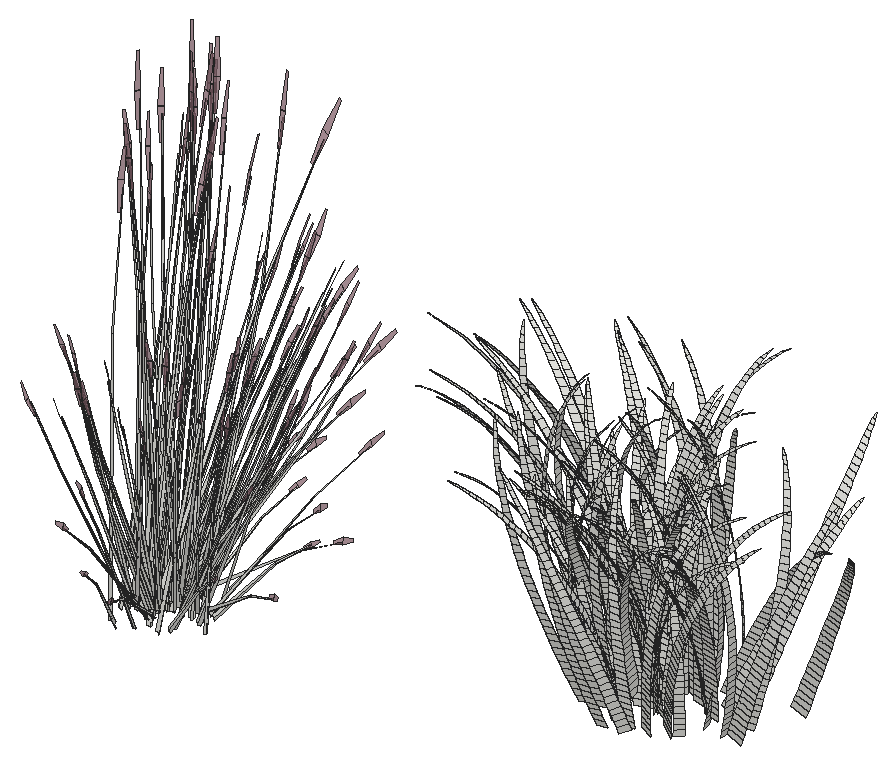
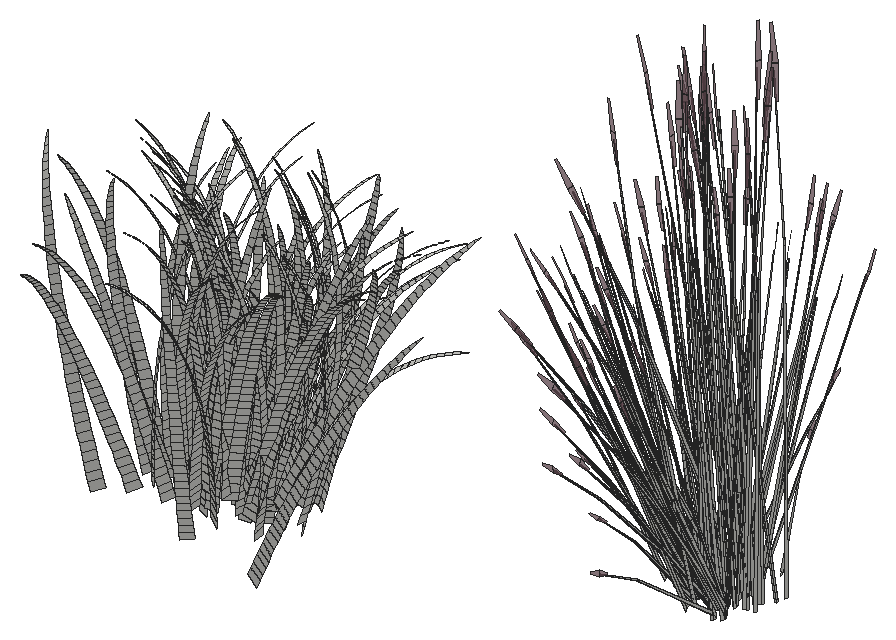
# SketchUp Ruby script. Lengths in inches.
U = 1.inch
M = Sketchup.active_model
def pt(a) = Geom::Point3d.new(a.map { |v| v * U })
def face(e, loops, mat)
  f = e.add_face(loops[0].map { |a| pt(a) })
  loops[1..].each { |l| e.add_face(l.map { |a| pt(a) }).erase! }
  f.material = f.back_material = mat if mat
  f
end
# faces: each face lists its corners as indices into pts; further lists are holes
def faces(e, pts, list, mat = nil) = list.each { |f| face(e, (f[0].is_a?(Array) ? f : [f]).map { |l| l.map { |i| pts[i] } }, mat) }
# xy, xz, yz: faces in a plane at the given z, y or x. An outline is a flat list of corners, or four numbers for a rectangle; further outlines are holes
def ring(l) = l.size == 4 ? [[l[0], l[1]], [l[2], l[1]], [l[2], l[3]], [l[0], l[3]]] : l.each_slice(2).to_a
def flat(e, list, mat, &to3) = list.each { |f| face(e, (f[0].is_a?(Array) ? f : [f]).map { |l| ring(l).map { |u, v| to3.(u, v) } }, mat) }
def xy(e, z, list, mat = nil) = flat(e, list, mat) { |x, y| [x, y, z] }
def xz(e, y, list, mat = nil) = flat(e, list, mat) { |x, z| [x, y, z] }
def yz(e, x, list, mat = nil) = flat(e, list, mat) { |y, z| [x, y, z] }
def lines(e, pts, list) = list.each { |a, b| e.add_line(pt(pts[a]), pt(pts[b])) }
# prism: a flat outline (further loops are holes) pulled along v
def prism(e, loops, v, mat = nil)
  f = face(e, loops, mat); d = Geom::Vector3d.new(v.map { |x| x * U })
  f.pushpull(f.normal.samedirection?(d) ? d.length : -d.length)
end
def box(e, o, s, mat = nil) = prism(e, [[o, [o[0] + s[0], o[1], o[2]], [o[0] + s[0], o[1] + s[1], o[2]], [o[0], o[1] + s[1], o[2]]]], [0, 0, s[2]], mat)
def at(x, y, z, deg = 0) = Geom::Transformation.translation(pt([x, y, z])) * Geom::Transformation.rotation(ORIGIN, Z_AXIS, deg.degrees)
def axes(o, x, y, z) = Geom::Transformation.new([*x, 0, *y, 0, *z, 0, *pt(o).to_a, 1])
def part(name) = M.definitions.add(name)
# library, detail: a bought-in or finely detailed component or shape, given as its bounding box
def library(name, o, s) = part(name).tap { |d| box(d.entities, o, s) }
def detail(e, o, s) = box(e.add_group.entities, o, s)
def put(e, d, t, mat = nil) = e.add_instance(d, t).tap { |i| i.material = mat if mat }
def group(e, t, mat = nil) = e.add_group.tap { |g| g.transformation = t; g.material = mat if mat }.entities
root = M.entities
M.materials.add("LightPink_Translucent").color = [144, 107, 117]
M.materials["LightPink_Translucent"].alpha = 0.75
c1 = part("blade")
p = [[2.15,0.21,22],[0,0.17,0],[0.09,0.45,0],[2.18,0.31,22],[2.29,0.31,22],[0.38,0.45,0],
  [2.48,0.24,33],[2.49,0.24,33],[2.48,0.22,33]]
faces(c1.entities,p,[[0,1,2,3],[4,5,2,3],[6,3,4,7],[8,0,3,6]])
c2 = part("seeds")
p = [[0.3,-0.1,1.38],[-0.01,-0.03,1.59],[-0.01,-0.03,0.03],[0.14,-0.07,-0.07],[0.29,-0.03,3],[0.15,0.01,3.11]]
faces(c2.entities,p,[[0,1,2,3],[1,0,4,5]],"LightPink_Translucent")
c3 = part("blade with seeds")
put(c3.entities,c1,at(0,0,0))
put(c3.entities,c2,axes([2.4,0.25,30.99],[1.5799,-0.05474,1.17369],[-0.12525,1.92788,0.29478],[-0.07173,-0.02425,1.56792]))
c4 = part("fur_instance\#8")
p = [[-0.25,1.49,0.03],[0.25,-1.49,-0.03],[0.44,-1.47,1.51],[-0.05,1.47,1.57],[0.65,-1.44,3.05],[0.16,1.45,3.11],
  [0.86,-1.42,4.59],[0.38,1.44,4.65],[1.1,-1.39,6.13],[0.62,1.43,6.18],[1.34,-1.35,7.66],[0.875,1.42,7.72],
  [1.6,-1.32,9.19],[1.14,1.41,9.25],[1.88,-1.28,10.72],[1.43,1.41,10.78],[2.18,-1.24,12.25],[1.73,1.41,12.3],
  [2.49,-1.19,13.77],[2.05,1.41,13.82],[2.83,-1.15,15.29],[2.4,1.41,15.34],[3.18,-1.09,16.8],[2.76,1.42,16.85],
  [3.56,-1.03,18.31],[3.14,1.43,18.35],[3.96,-0.97,19.81],[3.55,1.44,19.85],[4.38,-0.91,21.3],[3.99,1.46,21.35],
  [4.84,-0.83,22.78],[4.45,1.48,22.83],[5.32,-0.76,24.26],[4.93,1.51,24.31],[5.82,-0.67,25.73],[5.45,1.54,25.77],
  [6.36,-0.59,27.18],[6,1.57,27.23],[6.93,-0.49,28.625],[6.58,1.61,28.67],[7.54,-0.39,30.05],[7.19,1.66,30.1],
  [8.18,-0.28,31.47],[7.84,1.71,31.51],[8.85,-0.16,32.86],[8.53,1.77,32.9],[9.57,-0.04,34.24],[9.25,1.83,34.27],
  [10.32,0.09,35.59],[10.02,1.9,35.625],[11.12,0.23,36.92],[10.82,1.97,36.95],[11.95,0.38,38.22],[11.67,2.06,38.25],
  [12.84,0.54,39.49],[12.57,2.14,39.52],[13.76,0.71,40.73],[13.51,2.24,40.76],[14.73,0.89,41.93],[14.49,2.34,41.95],
  [15.75,1.08,43.09],[15.52,2.45,43.11],[16.82,1.28,44.2],[16.6,2.5625,44.23],[17.93,1.5,45.27],[17.73,2.68,45.29],
  [19.08,1.73,46.28],[18.9,2.81,46.3],[20.29,1.97,47.24],[20.125,2.93,47.26],[21.53,2.22,48.13],[21.39,3.0625,48.15],
  [22.82,2.5,48.96],[22.7,3.1875,48.98],[24.14,2.8125,49.72],[24.06,3.3,49.73],[25.48,3.27,50.41]]
faces(c4.entities,p,[[0,1,2,3],[3,2,4,5],[5,4,6,7],[7,6,8,9],[9,8,10,11],[11,10,12,13],[13,12,14,15],[15,14,16,17],
  [17,16,18,19],[19,18,20,21],[21,20,22,23],[23,22,24,25],[25,24,26,27],[27,26,28,29],[29,28,30,31],[31,30,32,33],
  [33,32,34,35],[35,34,36,37],[37,36,38,39],[39,38,40,41],[41,40,42,43],[43,42,44,45],[45,44,46,47],[47,46,48,49],
  [49,48,50,51],[51,50,52,53],[53,52,54,55],[55,54,56,57],[57,56,58,59],[59,58,60,61],[61,60,62,63],[63,62,64,65],
  [65,64,66,67],[67,66,68,69],[69,68,70,71],[71,70,72,73],[73,72,74,75],[75,74,76]])
put(root,c3,axes([255.16,15.57,16.52],[0.29095,-0.70883,-0.30711],[0.84882,0.20674,0.39649],[-0.07783,-0.28538,0.75865]))
put(root,c3,axes([253.74,19.4,14.64],[0.41959,1.03069,0.39679],[-1.19889,0.35841,0.15571],[0.01465,-0.18939,1.37763]))
put(root,c3,axes([254.75,21.94,14.5],[-0.31488,-0.79467,0],[0.89916,-0.27829,0],[0,0,1.33873]))
put(root,c3,axes([253.8125,23.9,16.52],[-0.29095,0.70883,-0.30711],[-0.84882,-0.20674,0.39649],[0.07783,0.28538,0.75865]))
put(root,c3,axes([255.52,15.67,16.69],[0.71112,-0.31326,0.05576],[0.34807,0.57124,0.43899],[-0.06868,-0.25181,0.6694]))
put(root,c3,axes([253.21,25.16,16.68],[0.12233,0.14843,1.51715],[0.98723,0.05831,-0.23994],[0.09927,0.32734,0.12168]))
put(root,c3,axes([257.87,19.87,14.74],[-0.75824,-0.6714,0.153],[0.76412,-0.65122,0.30427],[-0.08374,0.13711,1.39107]))
put(root,c3,axes([255.25,19.48,14.5],[0,-1.06651,0],[1.20676,0,0],[0,0,1.55627]))
put(root,c3,axes([255.27,15.73,16.7],[0.95095,0.24097,0.41629],[-0.32517,0.79222,0.34325],[-0.05715,-0.31154,0.8614]))
put(root,c3,axes([254.13,19.68,14.7],[1.08738,0.44674,0.20869],[-0.52332,0.92827,0.43363],[0,-0.21398,1.39225]))
put(root,c3,axes([255.86,19.91,14.58],[0,1.06599,-0.04888],[-1.20676,0,0],[0,0.0335,1.5555]))
put(root,c3,axes([253.78,19.05,14.95],[-1.04798,0.0569,0.38798],[-0.09477,-0.94451,-0.18672],[0.18761,-0.09573,1.2457]))
put(root,c3,axes([253.72,23.15,16.97],[0.29095,-0.70883,0.30711],[0.84882,0.20674,-0.39649],[0.07783,0.28538,0.75865]))
put(root,c3,axes([253.29,17.43,14.74],[-0.27879,0.91605,0.153],[-1.02019,-0.25923,0.30427],[0.17623,-0.00446,1.39107]))
put(root,c3,axes([255.28,21.97,14.58],[0.41959,1.05891,-0.05214],[-1.19889,0.37105,0],[0.01465,0.03698,1.49311]))
put(root,c3,axes([252.79,16.3,14.65],[-0.60338,-0.92363,0],[1.00947,-0.51509,-0.44755],[0.22991,-0.11731,1.41973]))
put(root,c3,axes([253.9,23.26,16.91],[0.46061,0.74947,-0.61612],[-0.94816,0.41768,0.07435],[0.10771,0.36212,0.87156]))
put(root,c3,axes([258.74,20.58,14.5],[-1.20616,-0.00737,-0.04316],[0,-1.03017,0.43311],[-0.03791,0.23451,1.37325]))
put(root,c3,axes([256.375,17.48,14.74],[-1.03704,0.24464,0.153],[-0.25607,-0.91045,0.30427],[0.09249,0.13265,1.39107]))
put(root,c3,axes([255.32,14.07,14.99],[0.1238,0.53749,0.99609],[-0.68678,-0.29769,0.73186],[0.0739,-0.27521,0.2194]))
put(root,c3,axes([254.86,25.68,17.49],[0.6669,-0.52879,-0.05626],[0.61107,0.57914,-0.2551],[0.04302,0.1641,0.84141]))
put(root,c3,axes([254.68,18.8125,14.64],[-0.80019,0.83649,0.39679],[-0.95065,-0.7384,0.15571],[0.19291,-0.08348,1.37763]))
put(root,c3,axes([256.05,20.13,14.51],[0.67366,0.59537,0],[-0.67366,0.59537,0],[0,0,1.4679]))
put(root,c3,axes([256.04,19.43,14.95],[0.46824,-0.83055,0.38798],[0.97292,0.39972,-0.18672],[0,0.19146,1.2457]))
put(root,c3,axes([255.63,22.32,14.5],[0.97292,0.41382,0],[-0.46824,0.85985,0],[0,0,1.51723]))
put(root,c3,axes([254.24,23.41,16.65],[0.94868,0.23106,-0.44314],[-0.32517,0.79222,-0.34325],[0.08699,0.31896,0.8479]))
put(root,c3,axes([253.43,23.45,16.96],[0.94439,-0.42914,-0.10546],[0.46409,0.76165,-0.58532],[0.1246,0.32096,0.88939]))
put(root,c3,axes([255.72,19.24,14.66],[-1.21977,-0.1942,0.42666],[0.24824,-1.0968,0.16743],[0.17826,0.10591,1.48132]))
put(root,c3,axes([258.26,14.95,16.68],[-0.09801,0.0704,1.5383],[-0.96025,-0.23753,-0.14535],[-0.03476,-0.30724,0.27223]))
put(root,c3,axes([257.5,16.98,16.96],[-1.06065,-0.04567,-0.10546],[0.02899,-0.86469,-0.58532],[0.07368,-0.33302,0.88939]))
put(root,c3,axes([256.07,19.72,14.51],[1.07973,0,0],[0,0.95425,0],[0,0,1.54717]))
put(root,c3,axes([257.09,17.11,16.97],[-0.65298,0.48529,0.30711],[-0.61814,-0.55413,-0.39649],[0.09405,-0.28154,0.75865]))
put(root,c3,axes([255.03,18.67,14.95],[-0.57975,-0.77365,0.38798],[0.87815,-0.54479,-0.18672],[0.18761,0.09573,1.2457]))
put(root,c3,axes([256.44,19.625,14.86],[0.89916,-0.26881,0.12557],[0.31488,0.76759,-0.35857],[0,0.16893,1.09915]))
put(root,c3,axes([256.78,16.66,16.65],[-0.69086,-0.61932,-0.44314],[0.72981,-0.54239,-0.34325],[0.10512,-0.31467,0.8479]))
put(root,c3,axes([256.33,15.56,14.84],[-0.27432,0.18657,1.24013],[-0.82156,-0.32655,-0.2667],[0.15229,-0.40611,0.53022]))
put(root,c3,axes([258.49,19.9,14.74],[0,-0.92173,0.43058],[1.07973,0,0],[0,0.20993,1.3659]))
put(root,c3,axes([256.07,23.54,16.7],[-0.95987,0.21153,0.41629],[-0.16659,-0.82977,0.34325],[0.22575,0.24455,0.8614]))
put(root,c3,axes([255.89,23.71,16.69],[-0.43862,0.58553,0.05576],[-0.62461,-0.3409,0.43899],[0.20194,0.18773,0.6694]))
put(root,c3,axes([254.78,21.78,15.95],[-0.2206,-0.29594,1.4862],[1.01938,-0.24915,0.12017],[0.23039,0.4646,0.63534]))
put(root,c3,axes([255.42,18.45,14.86],[0.18618,-0.8226,0.12557],[0.90961,0.14279,-0.35857],[0.16554,0.08447,1.09915]))
put(root,c3,axes([256.71,17.02,14.74],[-0.90321,-0.46087,0.43058],[0.53987,-0.8264,0],[0.20571,0.10497,1.3659]))
put(root,c3,axes([256.99,16.9375,16.91],[0.02511,-0.8526,-0.61612],[1.05743,0.05726,0.07435],[0.11159,-0.3612,0.87156]))
put(root,c3,axes([255.75,23.04,16.97],[-0.14905,-0.74243,0.30711],[0.85206,-0.19604,-0.39649],[0.22886,0.21276,0.75865]))
put(root,c3,axes([256.33,18.77,16.47],[-0.83393,-0.47892,1.19921],[0.88055,-0.74565,0.51742],[0.26905,0.44936,1.15915]))
put(root,c3,axes([257.43,16.43,16.52],[0.65298,-0.48529,-0.30711],[0.61814,0.55413,0.39649],[0.09405,-0.28154,0.75865]))
put(root,c3,axes([254.92,24.08,16.68],[0.00286,-0.11159,1.5383],[0.82704,-0.49234,-0.14535],[0.28727,0.17573,0.27223]))
put(root,c3,axes([257.68,16.67,16.69],[0.79307,0.04295,0.05576],[-0.02174,0.64852,0.43899],[0.08299,-0.24842,0.6694]))
put(root,c3,axes([257.59,22.66,14.99],[-0.54338,-0.26503,0.99609],[0.70163,-0.26929,0.73186],[0.18925,0.22811,0.2194]))
put(root,c3,axes([255.65,22.38,14.84],[0.01703,-0.30555,1.24013],[0.81385,-0.34129,-0.2667],[0.25124,0.36571,0.53022]))
put(root,c3,axes([258.47,15.61,16.68],[-0.00932,-0.18345,1.51715],[-0.78682,-0.53019,-0.23994],[0.12165,-0.32139,0.12168]))
put(root,c3,axes([257.43,16.61,16.7],[0.68722,0.6289,0.41629],[-0.72981,0.54239,0.34325],[0.12676,-0.29506,0.8614]))
put(root,c3,axes([259.23,20.05,14.65],[1.20676,0,0],[0,1.03017,-0.44755],[0,0.23463,1.41973]))
put(root,c3,axes([257.67,23.87,14.91],[-0.61887,-0.02891,0.9111],[0.4087,-0.61397,0.50304],[0.24448,0.21813,0.71468]))
put(root,c3,axes([258.22,18.61,16.97],[-0.84006,0.13173,0.30711],[-0.22182,-0.75304,-0.39649],[0.24073,-0.20226,0.75865]))
put(root,c3,axes([255.8,16.51,15.95],[-0.17969,0.31682,1.4862],[-0.75383,-0.65564,0.12017],[0.34007,-0.40863,0.63534]))
put(root,c3,axes([255.68,23.42,16.96],[0.57508,-0.78896,-0.10546],[0.83282,0.45453,-0.58532],[0.28949,0.2229,0.88939]))
put(root,c3,axes([258.66,18.68,16.96],[-0.89271,-0.50824,-0.10546],[0.5143,-0.73603,-0.58532],[0.25221,-0.25585,0.88939]))
put(root,c3,axes([256.36,23.03,16.65],[0.95231,-0.21911,-0.44314],[0.16659,0.82977,-0.34325],[0.25579,0.23779,0.8479]))
put(root,c3,axes([257.23,16.54,14.65],[0.60338,-0.92363,0],[1.00947,0.51509,-0.44755],[0.22991,0.11731,1.41973]))
put(root,c3,axes([257.45,22.03,16.97],[-0.54911,-0.5771,0.30711],[0.627,-0.5463,-0.39649],[0.31857,0.08312,0.75865]))
put(root,c3,axes([257.95,22.56,16.69],[-0.0486,0.70091,0.05576],[-0.7338,-0.01922,0.43899],[0.28109,0.07334,0.6694]))
put(root,c3,axes([258.02,22.33,16.7],[-0.7116,0.60735,0.41629],[-0.61371,-0.64499,0.34325],[0.33386,0.11203,0.8614]))
put(root,c3,axes([258.21,18.08,16.65],[-0.24792,-0.84163,-0.44314],[0.93889,-0.14723,-0.34325],[0.26906,-0.22606,0.8479]))
put(root,c3,axes([259.87,22.42,16],[-0.18471,-0.77483,-0.03028],[0.87303,-0.17813,-0.13729],[0.18231,0.04912,0.45285]))
put(root,c3,axes([258.36,20.41,16.97],[-0.80204,-0.25713,0.30711],[0.23393,-0.75017,-0.39649],[0.32291,-0.06879,0.75865]))
put(root,c3,axes([260.74,19.41,14.55],[-0.59832,-0.5894,-0.05626],[0.65529,-0.54005,-0.2551],[0.18568,-0.03802,0.84141]))
put(root,c3,axes([259.37,16.41,14.99],[-0.32145,0.46921,0.99609],[-0.2763,-0.6304,0.73186],[0.26549,-0.15796,0.2194]))
put(root,c3,axes([258.98,18.49,16.69],[0.66253,0.38765,0.05576],[-0.38573,0.55202,0.43899],[0.21241,-0.17847,0.6694]))
put(root,c3,axes([258.8,18.33,16.7],[0.23935,0.84832,0.41629],[-0.93889,0.14723,0.34325],[0.27671,-0.19951,0.8614]))
put(root,c3,axes([256.26,20.86,15.95],[-0.35848,-0.15881,1.4862],[0.74185,-0.66622,0.12017],[0.46237,0.30054,0.63534]))
put(root,c3,axes([260.86,18.46,16.68],[-0.12605,-0.007,1.5383],[-0.52344,-0.75009,-0.14535],[0.21021,-0.24663,0.27223]))
put(root,c3,axes([258.91,18.17,16.52],[0.84006,-0.13173,-0.30711],[0.22182,0.75304,0.39649],[0.24073,-0.20226,0.75865]))
put(root,c3,axes([258.24,18.42,16.91],[0.50411,-0.72728,-0.61612],[0.88337,0.51686,0.07435],[0.30099,-0.2635,0.87156]))
put(root,c3,axes([259.08,20.65,16.69],[0.35445,0.62848,0.05576],[-0.64636,0.30762,0.43899],[0.28492,-0.06069,0.6694]))
put(root,c3,axes([258.23,22.33,16.52],[0.54911,0.5771,-0.30711],[-0.627,0.5463,0.39649],[0.31857,0.08312,0.75865]))
put(root,c3,axes([257.6,22.4,16.96],[0.05167,-0.93738,-0.10546],[0.97839,0.02562,-0.58532],[0.37682,0.06511,0.88939]))
put(root,c3,axes([258.69,20.67,16.96],[-0.48557,-0.83463,-0.10546],[0.86181,-0.41016,-0.58532],[0.36317,-0.11012,0.88939]))
put(root,c3,axes([259.01,20.42,16.7],[-0.27266,0.84043,0.41629],[-0.89639,-0.28738,0.34325],[0.35251,-0.05051,0.8614]))
put(root,c3,axes([258.45,21.84,16.68],[0.20703,-0.01559,1.51715],[0.56785,-0.71609,-0.23994],[0.36824,0.09453,0.12168]))
put(root,c3,axes([258.65,19.95,16.65],[0.26145,-0.83843,-0.44314],[0.89639,0.28738,-0.34325],[0.3609,-0.07688,0.8479]))
put(root,c3,axes([260.9,20.48,14.99],[-0.59628,0.15217,0.99609],[0.28067,-0.62889,0.73186],[0.31633,0.04303,0.2194]))
put(root,c3,axes([258.97,17.75,14.84],[-0.34476,-0.0273,1.24013],[-0.3532,-0.73238,-0.2667],[0.42354,-0.20718,0.53022]))
put(root,c3,axes([259.2,20.33,16.52],[0.80204,0.25713,-0.30711],[-0.23393,0.75017,0.39649],[0.32291,-0.06879,0.75865]))
put(root,c3,axes([257.65,21.95,16.91],[0.96472,0.02219,-0.61612],[-0.06479,0.93454,0.07435],[0.4087,0.09862,0.87156]))
put(root,c3,axes([259.61,20.1875,14.3125],[-0.62157,0.11062,1.22783],[-0.09894,-0.88048,0.07028],[0.43535,-0.13327,0.69868]))
put(root,c3,axes([260.625,23.15,16.68],[-0.08727,-0.08069,1.5383],[0.19089,-0.86497,-0.14535],[0.34373,-0.05526,0.27223]))
put(root,c3,axes([257.01,19.4,15.95],[-0.4003,0.02088,1.4862],[0.26555,-0.90478,0.12017],[0.57046,0.05596,0.63534]))
put(root,c3,axes([258.48,20.25,16.91],[0.84803,-0.40708,-0.61612],[0.4726,0.83797,0.07435],[0.40974,-0.09519,0.87156]))
put(root,c3,axes([261.33,19.36,16.68],[0.13392,-0.1404,1.51715],[-0.17141,-0.86122,-0.23994],[0.33602,-0.16329,0.12168]))
put(root,c3,axes([259.78,21.49,14.84],[-0.23242,-0.2267,1.24013],[0.30241,-0.74993,-0.2667],[0.47025,0.10159,0.53022]))
put(root,c4,axes([290.68,39.44,17.7],[-0.50763,-0.01588,-0.11604],[0.07324,-0.38696,0.09957],[-0.14007,-0.01726,0.52324]))
put(root,c4,axes([289.93,42.65,15],[-0.24797,-0.31039,0.07255],[0.41295,-0.20225,0.23078],[-0.1793,0.05655,0.46816]))
put(root,c4,axes([292.19,36.28,18.52],[-0.19293,-0.32428,-0.06942],[0.46679,-0.19975,0.14476],[-0.16878,-0.07561,0.52187]))
put(root,c4,axes([294.23,36.55,18.83],[-0.40343,0.27748,-0.04006],[-0.34183,-0.25952,-0.03577],[-0.06533,-0.08108,0.54363]))
put(root,c4,axes([291.69,33.64,17.58],[-0.02776,0.35202,0.0921],[-0.50219,0.05342,-0.13597],[-0.14228,-0.13593,0.51013]))
put(root,c4,axes([294.24,37.18,18.68],[-0.4054,0.27215,-0.04581],[-0.33526,-0.26485,-0.01486],[-0.05659,-0.068,0.54035]))
put(root,c4,axes([293.91,34.63,17.49],[-0.41183,-0.15887,-0.04901],[0.27293,-0.31592,0.01909],[-0.06226,-0.08242,0.50785]))
put(root,c4,axes([294.96,34.4375,18.54],[-0.49226,-0.08023,-0.05731],[0.17603,-0.35913,-0.02376],[-0.05781,-0.10803,0.5357]))
put(root,c4,axes([296.04,34.23,18.59],[-0.4945,0.16018,-0.01115],[-0.17276,-0.32714,-0.06388],[-0.04389,-0.11924,0.53502]))
put(root,c4,axes([294.97,31.77,17.03],[-0.22789,0.30866,0.07999],[-0.42694,-0.09296,-0.13611],[-0.0957,-0.15962,0.48053]))
put(root,c4,axes([296.24,31.78,16.0625],[-0.34072,-0.1747,-0.05326],[0.29244,-0.26338,-0.00145],[-0.04965,-0.09279,0.4601]))
put(root,c4,axes([294.4,37.51,17.26],[-0.0622,-0.3553,0.08513],[0.48228,-0.079,0.11308],[-0.11283,-0.00228,0.49186]))
put(root,c4,axes([297.29,34.57,17.78],[-0.39363,-0.18552,-0.01372],[0.29927,-0.30535,0.04069],[-0.04685,-0.05915,0.50744]))
put(root,c4,axes([294.52,28.88,15.24],[-0.00016,0.26749,0.22995],[-0.47166,0.07885,-0.08309],[-0.1045,-0.2152,0.43076]))
put(root,c4,axes([296.59,37.38,18.26],[-0.26668,0.33554,-0.04082],[-0.44054,-0.16095,0.00169],[-0.03189,-0.05514,0.52743]))
put(root,c4,axes([295.42,32.99,16.6875],[-0.10805,0.33126,0.00833],[-0.45532,-0.03693,-0.05128],[-0.05831,-0.0845,0.48072]))
put(root,c4,axes([290.19,35.64,17.47],[0.49358,-0.11129,0.14866],[0.06221,0.35262,0.05998],[-0.16388,-0.09555,0.51254]))
put(root,c4,axes([298.27,30.06,16.26],[-0.46056,-0.04626,-0.0143],[0.11427,-0.29372,-0.1523],[0.01117,-0.17712,0.462]))
put(root,c4,axes([298.51,39.88,17.77],[-0.47274,0.18817,-0.02801],[-0.21717,-0.32936,0.14037],[0.0203,0.01491,0.51426]))
put(root,c4,axes([295.86,32.39,15.72],[-0.09622,0.31097,-0.00039],[-0.42605,-0.03207,-0.0465],[-0.05504,-0.07286,0.44897]))
put(root,c4,axes([297.75,37.41,17.96],[-0.31952,0.3051,-0.0298],[-0.39525,-0.20368,0.02449],[-0.01218,-0.05332,0.51983]))
put(root,c4,axes([291.03,32.06,16.99],[0.43281,0.12176,0.16061],[-0.27188,0.32921,0.04582],[-0.12478,-0.15481,0.51294]))
put(root,c4,axes([291.76,33.64,15.16],[0.40575,0.06024,0.13134],[-0.14648,0.31966,-0.03937],[-0.14415,-0.06458,0.44572]))
put(root,c4,axes([298.89,29.38,14.71],[-0.38894,0.10997,0.02117],[-0.12343,-0.25799,-0.04659],[-0.00409,-0.09941,0.41525]))
put(root,c4,axes([296.9,32.44,17.02],[-0.14716,0.32508,0.04733],[-0.456,-0.06503,-0.03692],[-0.03204,-0.11272,0.4887]))
put(root,c4,axes([292.54,34.8125,15.98],[0.44324,-0.00034,0.13389],[-0.06145,0.33975,-0.03971],[-0.1458,-0.04824,0.46189]))
put(root,c4,axes([296.82,28.42,15.74],[-0.08868,0.28043,0.25739],[-0.50846,-0.00649,-0.04871],[-0.01877,-0.25127,0.46021]))
put(root,c4,axes([296.89,34.05,16.41],[-0.05213,0.33127,-0.0306],[-0.45538,-0.00449,-0.02236],[-0.03636,-0.0514,0.4699]))
put(root,c4,axes([300.03,32.34,15.2],[-0.4142,0.07823,0.02606],[-0.07608,-0.29206,0.02381],[0.01891,-0.05531,0.43077]))
put(root,c4,axes([297.56,33.73,15.3],[-0.14518,-0.28229,0.10171],[0.40006,-0.1299,0.05907],[-0.03188,0.01644,0.42147]))
put(root,c4,axes([297.27,27.77,14.35],[0.00782,0.23498,0.21816],[-0.43216,0.05865,-0.03529],[-0.05593,-0.20575,0.38839]))
put(root,c4,axes([297.9375,28.99,14.57],[-0.05897,0.25645,0.12335],[-0.39967,0.00165,-0.04398],[-0.03657,-0.14736,0.39475]))
put(root,c4,axes([293.72,32.25,16.57],[0.45071,0.01134,0.13895],[-0.11047,0.32832,0.06043],[-0.13128,-0.12541,0.47068]))
put(root,c4,axes([299.86,27.68,14.74],[-0.32391,0.20212,0.20097],[-0.35191,-0.16271,-0.13597],[0.0269,-0.23384,0.42704]))
put(root,c4,axes([300.5,34.86,15.46],[-0.42909,0.09695,0.05136],[-0.09534,-0.30893,0.11238],[0.06344,-0.00492,0.43826]))
put(root,c4,axes([293.78,37.06,15.4],[0.43774,-0.10692,0.11225],[0.1037,0.31929,-0.06742],[-0.10438,-0.00211,0.45502]))
put(root,c4,axes([300.6,31.06,15.65],[-0.36297,-0.15414,0.01625],[0.24681,-0.26586,-0.04633],[0.02784,-0.09168,0.44826]))
put(root,c4,axes([296.13,33.01,14.21],[0.24527,-0.24268,0.11275],[0.30329,0.16231,0.01328],[-0.09051,-0.00183,0.39453]))
put(root,c4,axes([300.87,31.16,16.66],[-0.45745,-0.0815,0.06069],[0.12733,-0.30278,-0.13947],[0.08434,-0.15918,0.4705]))
put(root,c4,axes([300.88,38.31,17.7],[-0.40313,0.25423,-0.0016],[-0.31186,-0.27626,0.14327],[0.07356,-0.00571,0.50817]))
put(root,c4,axes([299.39,30.38,15.89],[-0.13723,0.3021,0.05577],[-0.42854,-0.06787,-0.00187],[0.00387,-0.10857,0.45799]))
put(root,c4,axes([295.02,30.11,15.15],[0.42424,-0.02112,0.10663],[-0.0575,0.29324,0.09056],[-0.10452,-0.12967,0.42964]))
put(root,c4,axes([297.87,33.79,14.21],[0.0172,-0.29324,0.11006],[0.40157,-0.01183,0.01497],[-0.03011,0.01552,0.39805]))
put(root,c4,axes([301.32,37.01,18.125],[-0.49269,0.10801,0.10975],[-0.11295,-0.36008,0.09876],[0.11457,-0.03866,0.51048]))
put(root,c4,axes([295.75,32.85,15.51],[0.25162,-0.27089,0.02967],[0.35002,0.15197,0.02917],[-0.05057,-0.06063,0.44306]))
put(root,c4,axes([298.27,37.84,16.82],[-0.0394,-0.35105,0.13413],[0.4872,-0.05905,0.00711],[-0.00865,0.01834,0.48291]))
put(root,c4,axes([295.27,41.27,18.15],[0.39799,0.23409,-0.0497],[-0.35236,0.31259,-0.14016],[-0.06959,0.01695,0.52915]))
put(root,c4,axes([300.54,31.6875,14.9],[-0.2469,-0.22146,0.03004],[0.32926,-0.1945,-0.02031],[0.02337,-0.05884,0.42108]))
put(root,c4,axes([300.68,32.06,17.42],[-0.3835,-0.20198,0.00054],[0.30916,-0.25497,-0.15778],[0.08749,-0.16513,0.48809]))
put(root,c4,axes([296.62,30.21,14.375],[0.2699,0.17584,0.04376],[-0.28369,0.21445,-0.01082],[-0.04675,-0.07597,0.4018]))
put(root,c4,axes([294.78,30.72,16.59],[0.46516,0.04499,0.10179],[-0.15491,0.31457,0.12274],[-0.07152,-0.17186,0.48232]))
put(root,c4,axes([300.65,36,14.91],[-0.25391,-0.24487,0.1199],[0.35833,-0.20844,0.02136],[0.04111,0.00539,0.43554]))
put(root,c4,axes([299.14,32.71,15.25],[-0.06686,-0.29524,0.0306],[0.41712,-0.07371,-0.01175],[0.00571,-0.04792,0.43193]))
put(root,c4,axes([294.04,35.34,18.51],[0.49909,-0.15056,0.0447],[0.15178,0.33969,0.03683],[-0.065,-0.09419,0.53587]))
put(root,c4,axes([298.63,33.83,15.42],[0.00943,-0.30977,0.03264],[0.43011,-0.0215,-0.00098],[-0.01031,-0.04514,0.44002]))
put(root,c4,axes([297.52,29.08,16.22],[0.18377,0.27757,0.15258],[-0.46804,0.14989,0.05588],[-0.01683,-0.18723,0.48957]))
put(root,c4,axes([295.84,31.77,17.45],[0.38506,-0.24657,-0.05064],[0.3168,0.20893,0.15406],[-0.07274,-0.17479,0.49054]))
put(root,c4,axes([300.12,32.69,17.64],[-0.03576,0.34789,0.05173],[-0.50087,0.00228,0.03007],[0.02066,-0.11511,0.51179]))
put(root,c4,axes([299.61,28.44,14.78],[-0.02199,0.27515,0.13478],[-0.4345,0.00114,0.03775],[0.03432,-0.15983,0.42499]))
put(root,c4,axes([300.6,32.375,15.45],[-0.0763,0.30565,0.00235],[-0.42363,-0.03176,0.0399],[0.02818,-0.06708,0.44047]))
put(root,c4,axes([299.62,31.31,15.44],[0.0066,0.29961,0.01973],[-0.42711,0.02592,0.04146],[0.02972,-0.08391,0.43662]))
put(root,c4,axes([296.46,31.55,14.77],[0.39392,0.03527,0.03594],[-0.09357,0.2896,-0.01536],[-0.0475,-0.05694,0.41614]))
put(root,c4,axes([298.1,38.55,18.98],[0.23236,0.33225,-0.04014],[-0.48314,0.19768,-0.00729],[-0.00257,-0.05784,0.54816]))
put(root,c4,axes([298.57,33.79,16.56],[0.15479,-0.32238,0.02323],[0.43589,0.08422,-0.02735],[0.00625,-0.05247,0.47294]))
put(root,c4,axes([303.13,33.7,17.13],[-0.42979,-0.15453,0.12454],[0.21947,-0.3163,-0.08244],[0.13305,-0.09644,0.49104]))
put(root,c4,axes([298.82,40.49,14.96],[0.17881,-0.325,0.20351],[0.44585,0.09863,-0.0895],[-0.00518,0.08565,0.43952]))
put(root,c4,axes([299.07,33.82,18.3],[0.18947,0.32214,0.03468],[-0.48115,0.15678,0.05093],[0.02127,-0.11854,0.52705]))
put(root,c4,axes([297.79,34.38,15.18],[0.36711,-0.18268,0.07793],[0.22046,0.25376,-0.08906],[-0.03208,0.01654,0.42408]))
put(root,c4,axes([303.5,30.4375,14.37],[-0.31479,0.18626,0.11902],[-0.25883,-0.22438,0.04673],[0.10912,-0.09793,0.41323]))
put(root,c4,axes([304.64,37.88,17.23],[-0.45166,-0.15139,0.1485],[0.23389,-0.34666,0.00439],[0.11529,-0.0389,0.51367]))
put(root,c4,axes([301.39,32.8,16.67],[0.02321,0.33175,0.01089],[-0.4716,0.04012,0.04727],[0.03399,-0.08645,0.48294]))
put(root,c4,axes([300.22,33.18,17.9375],[0.138,0.3338,0.03001],[-0.49096,0.12112,0.05086],[0.02745,-0.11217,0.5203]))
put(root,c4,axes([296.56,37.98,18.81],[0.52261,-0.09894,0.01657],[0.0883,0.36982,-0.0373],[-0.02292,-0.05546,0.5424]))
put(root,c4,axes([301.04,38.45,18.84],[-0.03206,-0.38843,0.10613],[0.52832,-0.05414,-0.10809],[0.1002,-0.02176,0.53115]))
put(root,c4,axes([299.45,33.17,18.33],[0.33717,0.25495,0.02672],[-0.39876,0.25463,0.05779],[0.01351,-0.12347,0.5318]))
put(root,c4,axes([301.32,31.66,16.3],[0.01124,0.31456,0.0667],[-0.45052,0.0071,0.12627],[0.1117,-0.12495,0.45411]))
put(root,c4,axes([299.375,33.56,16.16],[0.3065,-0.25628,0.00185],[0.33205,0.19993,-0.03621],[0.01369,-0.05484,0.46211]))
put(root,c4,axes([298.375,33.18,17.62],[0.49577,-0.02024,-0.01503],[-0.01468,0.34069,0.05964],[0.00426,-0.11967,0.50482]))
put(root,c4,axes([304.82,32.54,14.79],[-0.40072,0.01577,0.21122],[-0.01609,-0.32053,0.03805],[0.19799,-0.05795,0.40524]))
put(root,c4,axes([305.16,31.9,17.15],[-0.42933,-0.20545,0.08443],[0.25461,-0.26531,-0.25222],[0.19414,-0.19975,0.48041]))
put(root,c4,axes([298.39,34.24,18.67],[0.50354,0.07625,-0.00903],[-0.15271,0.35498,0.06351],[0.01361,-0.12441,0.53586]))
put(root,c4,axes([301.44,28.5625,14.87],[0.23508,0.23997,0.07058],[-0.37918,0.15814,0.12467],[0.05838,-0.15825,0.43852]))
put(root,c4,axes([299.67,31.86,16.25],[0.44136,0.05507,-0.02597],[-0.11205,0.31224,0.04588],[0.02451,-0.10015,0.46457]))
put(root,c4,axes([299.09,30.11,17.1],[0.49555,-0.1275,-0.07514],[0.16104,0.30057,0.15022],[0.01227,-0.19449,0.5073]))
put(root,c4,axes([307.07,32.32,14.9],[-0.41779,0.06908,0.23708],[-0.12585,-0.32343,-0.00178],[0.21241,-0.12582,0.43744]))
put(root,c4,axes([304.15,32.68,16.69],[-0.04795,-0.34418,-0.03233],[0.48122,-0.03593,-0.14824],[0.12949,-0.11621,0.49036]))
put(root,c4,axes([305.38,39.42,17.04],[-0.13733,0.37987,-0.07091],[-0.47203,-0.07363,0.24018],[0.1999,-0.00192,0.48306]))
put(root,c4,axes([305.37,32.54,15.96],[-0.04553,-0.33624,-0.03197],[0.47012,-0.03416,-0.1447],[0.12647,-0.1135,0.47892]))
put(root,c4,axes([301.1875,30.18,16.28],[0.47993,0.02108,-0.06101],[-0.04605,0.30986,0.1423],[0.06309,-0.17101,0.4739]))
put(root,c4,axes([301.74,31.92,16.89],[0.38033,0.19783,-0.03265],[-0.29076,0.25797,0.14918],[0.10401,-0.14804,0.47852]))
put(root,c4,axes([308.26,33.8,15.32],[-0.28524,0.26937,0.16985],[-0.35397,-0.23501,0.17849],[0.22861,-0.09933,0.45987]))
put(root,c4,axes([305.75,34.4,15.86],[0.02527,0.34976,-0.04562],[-0.43733,0.02339,0.22995],[0.21626,-0.0633,0.44264]))
put(root,c4,axes([303.57,28.83,15.52],[0.39282,0.20716,0.05352],[-0.32546,0.21595,0.25802],[0.11974,-0.23754,0.46819]))
put(root,c4,axes([303.61,36.97,15.62],[0.278,-0.29649,0.02543],[0.35647,0.18029,-0.22211],[0.15259,0.02475,0.43511]))
put(root,c4,axes([308.43,31.86,15.11],[0.07638,0.33967,0.08745],[-0.46737,0.01681,0.24022],[0.21187,-0.16565,0.46647]))
put(root,c4,axes([309.83,38.9,15.26],[0.07251,-0.3862,0.05218],[0.47979,0.03692,-0.2487],[0.22338,-0.03466,0.48518]))
